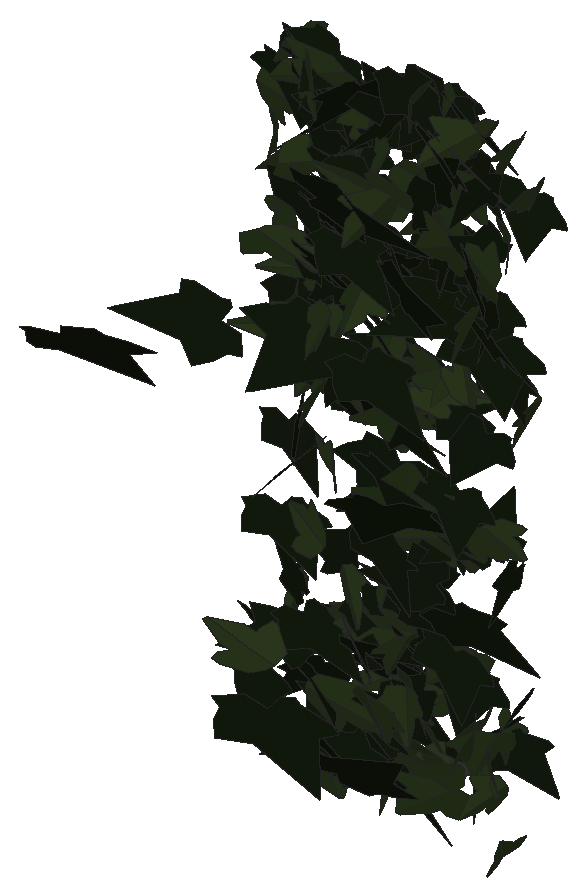
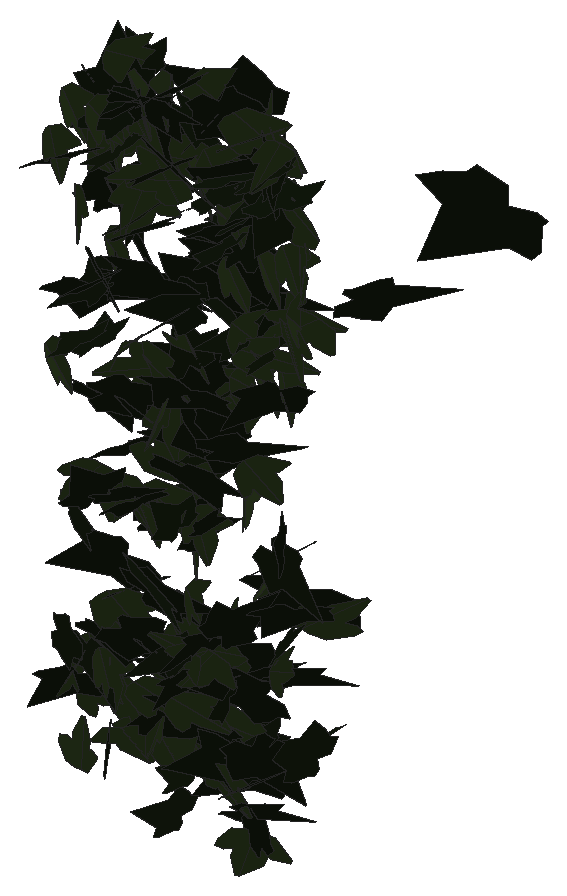
# SketchUp Ruby script. Lengths in millimetres.
U = 1.mm
M = Sketchup.active_model
def pt(a) = Geom::Point3d.new(a.map { |v| v * U })
def face(e, loops, mat)
  f = e.add_face(loops[0].map { |a| pt(a) })
  loops[1..].each { |l| e.add_face(l.map { |a| pt(a) }).erase! }
  f.material = f.back_material = mat if mat
  f
end
# faces: each face lists its corners as indices into pts; further lists are holes
def faces(e, pts, list, mat = nil) = list.each { |f| face(e, (f[0].is_a?(Array) ? f : [f]).map { |l| l.map { |i| pts[i] } }, mat) }
# xy, xz, yz: faces in a plane at the given z, y or x. An outline is a flat list of corners, or four numbers for a rectangle; further outlines are holes
def ring(l) = l.size == 4 ? [[l[0], l[1]], [l[2], l[1]], [l[2], l[3]], [l[0], l[3]]] : l.each_slice(2).to_a
def flat(e, list, mat, &to3) = list.each { |f| face(e, (f[0].is_a?(Array) ? f : [f]).map { |l| ring(l).map { |u, v| to3.(u, v) } }, mat) }
def xy(e, z, list, mat = nil) = flat(e, list, mat) { |x, y| [x, y, z] }
def xz(e, y, list, mat = nil) = flat(e, list, mat) { |x, z| [x, y, z] }
def yz(e, x, list, mat = nil) = flat(e, list, mat) { |y, z| [x, y, z] }
def lines(e, pts, list) = list.each { |a, b| e.add_line(pt(pts[a]), pt(pts[b])) }
# prism: a flat outline (further loops are holes) pulled along v
def prism(e, loops, v, mat = nil)
  f = face(e, loops, mat); d = Geom::Vector3d.new(v.map { |x| x * U })
  f.pushpull(f.normal.samedirection?(d) ? d.length : -d.length)
end
def box(e, o, s, mat = nil) = prism(e, [[o, [o[0] + s[0], o[1], o[2]], [o[0] + s[0], o[1] + s[1], o[2]], [o[0], o[1] + s[1], o[2]]]], [0, 0, s[2]], mat)
def at(x, y, z, deg = 0) = Geom::Transformation.translation(pt([x, y, z])) * Geom::Transformation.rotation(ORIGIN, Z_AXIS, deg.degrees)
def axes(o, x, y, z) = Geom::Transformation.new([*x, 0, *y, 0, *z, 0, *pt(o).to_a, 1])
def part(name) = M.definitions.add(name)
# library, detail: a bought-in or finely detailed component or shape, given as its bounding box
def library(name, o, s) = part(name).tap { |d| box(d.entities, o, s) }
def detail(e, o, s) = box(e.add_group.entities, o, s)
def put(e, d, t, mat = nil) = e.add_instance(d, t).tap { |i| i.material = mat if mat }
def group(e, t, mat = nil) = e.add_group.tap { |g| g.transformation = t; g.material = mat if mat }.entities
root = M.entities
M.materials.add("efeu1").color = [18, 25, 13]
M.materials.add("efeu2").color = [43, 57, 29]
c1 = part("ivyleaf_9")
p = [[39.1,54.8,31.7],[34.5,51.8,30.2],[-5.3,25.2,17.3],[-17.9,28.3,20.9],[-21.6,21.7,17],[-20.2,4.3,5.3],
  [-22.9,-0.3,2.5],[-17.1,-4,-0.6],[-2,-2.1,-1.2],[-0.7,-15.4,-10.1],[16.6,-22.3,-16.7],[21.1,-15.1,-12.5],
  [32.7,-10.7,-11],[46.1,-1.8,-6.6],[30.8,11.2,3.8]]
faces(c1.entities,p,[[0,1,2,3,4,5,6,7,8,9,10,11,12,13,14]],"efeu1")
c2 = part("ivyleaf_10")
p = [[0,12.8,-0.8],[-1.5,51.3,-10.9],[-4.9,51,-11.6],[-13.6,26.5,-7.3],[-13.2,15.9,-4.6],[-21.1,19.3,-7.2],
  [-29.5,16.3,-8.3],[-29.2,8.3,-6.2],[-19.7,-9.8,0.5],[-7.6,-13,4],[1,-12.2,5.8],[-0.4,51.1,-11.1],
  [-1.5,51.1,-10.9],[1,-12.4,5.9],[16.9,-12.4,3.5],[35.1,9.1,-5.1],[35,12.9,-6.1],[20.5,16.4,-4.9],
  [15.8,15,-3.8],[15.3,27.6,-7.1],[12.8,31.3,-7.8]]
faces(c2.entities,p,[[0,1,2,3,4,5,6,7,8,9,10],[11,12,0,13,14,15,16,17,18,19,20]],"efeu2")
put(root,c1,axes([3084.9,440.1,2359.8],[2.43652,0.60227,0.19081],[0.32002,0.09079,-1.41477],[-1.15902,1.29117,0.01048]))
put(root,c1,axes([3253.2,607.2,1847],[-0.95084,-0.69607,-0.93578],[1.0768,0.74556,-0.85664],[1.94097,-0.75461,0.01683]))
put(root,c1,axes([3139.5,650.3,2307],[-0.43713,-0.83768,-0.9062],[-0.15243,-0.9097,0.86121],[-2.34372,0.2154,0.11301]))
put(root,c1,axes([3401,666.2,2424.2],[0.21234,-0.26339,1.12095],[0.68031,-1.06264,-0.28526],[2.08323,0.37387,-0.0211]))
put(root,c1,axes([3288.6,659,2515.6],[1.23779,-0.49363,1.04714],[1.54799,-0.65984,-0.81622],[1.56783,1.04121,-0.02082]))
put(root,c2,axes([3362.4,672.8,2529.3],[-0.43007,-0.85809,0.7892],[0.0085,-0.80451,-0.87347],[2.21879,-0.16325,0.15632]))
put(root,c1,axes([3380.9,659.5,2140.2],[1.09267,0.78644,-0.62157],[-0.71114,-0.49678,-0.97368],[-1.7703,0.68496,0.00748]))
put(root,c1,axes([3299.5,679.7,1749.2],[2.29067,0.26504,-0.0966],[0.16641,0.05198,1.23201],[0.51044,-1.20634,0.03186]))
put(root,c2,axes([3175.6,683.9,1862.2],[0.67109,0.79349,0.70985],[-0.634,-0.628,0.86747],[1.92454,-0.48357,0.03824]))
put(root,c1,axes([3340.4,677.1,2306],[0.14442,-0.8753,-0.73036],[0.10422,0.73393,-0.87389],[2.16712,0.02304,0.0907]))
put(root,c1,axes([3302.2,682.8,2456.8],[0.32635,-0.95084,-0.60499],[-0.13617,0.60154,-0.96569],[2.14057,0.18323,0.03081]))
put(root,c2,axes([3265.3,688.2,2334.5],[0.98608,-1.04399,-0.01718],[-0.01274,0.01586,-1.16548],[1.98715,0.51816,0.00105]))
put(root,c1,axes([3257,706.1,2301.3],[-2.32839,-0.5287,0.1001],[-0.16005,-0.0577,-1.33262],[1.01152,-1.22614,0.01955]))
put(root,c2,axes([3216.5,722.5,2294.8],[0.46106,0.07581,-1.10045],[-1.9081,-0.4547,-0.25203],[-0.87544,1.03098,-0.03024]))
put(root,c2,axes([3227.8,728.4,2215.6],[0.4675,-1.1153,0.05987],[0.00274,-0.06099,-1.14197],[2.12569,0.24536,-0.0117]))
put(root,c1,axes([3392,747.8,2574.5],[-0.037,-0.57224,0.85225],[0.31829,-0.84278,-0.56207],[1.92762,0.12817,0.10917]))
put(root,c1,axes([3305.3,745.4,2033.4],[0.28687,-1.09674,0.2171],[0.11462,-0.21078,-1.10663],[2.12472,0.15945,0.03039]))
put(root,c2,axes([3281.5,742.7,2351.7],[0.43735,0.77284,-0.59729],[-0.4549,-0.55045,-0.80419],[-1.80243,0.32645,0.05803]))
put(root,c2,axes([3421.7,726,2470.2],[-1.05772,0.28526,0.81128],[-1.46021,0.27184,-0.62117],[-0.73928,-0.94506,0.0662]))
put(root,c1,axes([3388.1,745.4,2535.1],[-0.29941,0.45568,0.90404],[0.1623,-0.90567,0.47135],[1.91993,0.14762,0.10114]))
put(root,c1,axes([3440.8,755.8,2408.1],[-0.42729,0.1807,1.00874],[-0.3584,-1.02236,0.14123],[1.91719,-0.15084,0.25123]))
put(root,c1,axes([3168.2,753.6,2452.7],[0.57952,-1.00657,0.18188],[0.07841,-0.17754,-1.05155],[1.94514,0.30705,-0.0118]))
put(root,c2,axes([3414.6,763.7,2595.5],[-0.43005,-0.41598,0.99444],[-0.14831,-1.00709,-0.43898],[2.04616,-0.16043,0.17719]))
put(root,c2,axes([3315.3,751,2482.2],[-0.56727,0.07463,-1.10758],[-2.0923,0.13924,0.30523],[0.29308,1.1385,0.03528]))
put(root,c1,axes([3208.5,766.7,1710.9],[1.70196,-0.66762,-0.15371],[0.27114,-0.066,1.11553],[-1.27536,-0.90497,0.03204]))
put(root,c1,axes([3408.9,772.5,2553.5],[1.72321,-0.64183,-0.32418],[0.50025,-0.18977,1.10984],[-1.2738,-0.94281,-0.0027]))
put(root,c1,axes([3361.2,773.6,1981.8],[-0.52982,-0.10978,0.97763],[-1.44305,-0.62342,-0.28591],[1.19296,-0.80287,0.08833]))
put(root,c1,axes([3303.7,782.9,2087.5],[-0.72654,-0.62867,0.8567],[0.29997,-0.93373,-0.61496],[2,-0.08833,0.40345]))
put(root,c1,axes([3222.7,760.2,2394.3],[1.22867,-0.77965,-0.32909],[-0.29418,0.29831,-1.00997],[1.5835,0.66037,0.06771]))
put(root,c1,axes([3154.6,776.4,1838.7],[-1.21132,-0.29447,0.5931],[-0.9294,-0.34687,-0.69626],[0.85116,-0.79783,0.0838]))
put(root,c2,axes([3287.1,757.9,1803.1],[-1.50348,0.50222,0.00553],[-0.00919,0.0027,-0.9361],[-0.95584,-0.78999,0.00031]))
put(root,c1,axes([3216,782.5,2221.8],[-0.21759,-0.75041,0.67425],[-0.26801,-0.66005,-0.75848],[1.90119,-0.17893,-0.02976]))
put(root,c1,axes([3195,766,2422.5],[1.62596,-0.61914,0.39765],[0.6118,-0.23407,-1.05509],[1.25974,0.91281,-0.00084]))
put(root,c2,axes([3304.7,777.7,1715.9],[0.39413,-0.85,0.63633],[0.46084,-0.59343,-0.8715],[1.96756,0.30926,0.07665]))
put(root,c2,axes([3466.3,749.9,2432.6],[0.26733,-0.01361,1.16168],[-1.89132,0.60472,0.12725],[-1.14532,-1.00178,0.06103]))
put(root,c2,axes([3166.8,783.1,2592.8],[0.50539,-0.51544,0.98689],[1.33139,-0.71205,-0.56012],[1.64849,0.7331,0.14983]))
put(root,c1,axes([3440.1,776.5,2549.4],[-1.52417,0.39954,-0.55784],[0.96461,-0.2335,-0.89485],[-0.88029,-0.94764,-0.0147]))
put(root,c2,axes([3165.2,752.1,2483.1],[-0.21986,-0.19847,-1.04461],[1.00364,0.90173,-0.22964],[1.75725,-0.53985,0.00046]))
put(root,c2,axes([3425.5,762.8,1808.3],[0.22232,-1.01962,-0.54688],[0.076,0.55289,-1.02229],[2.20074,0.08391,0.09055]))
put(root,c1,axes([3098.4,777.6,1769.3],[0.54312,-1.01097,-0.18089],[-0.10777,0.17197,-1.05044],[1.95166,0.29083,-0.00766]))
put(root,c2,axes([3407.4,785.3,2345.9],[0.45786,-0.90348,0.49968],[0.32991,-0.47043,-0.93406],[1.93707,0.29368,0.04098]))
put(root,c2,axes([3439.1,792,1726.4],[-0.17974,-0.43705,0.83311],[0.02416,-0.83781,-0.43807],[1.79035,-0.03257,0.08955]))
put(root,c2,axes([3314.9,781.7,2071.8],[-1.7452,-0.72204,-0.07403],[-0.09923,-0.05344,1.1671],[-1.37783,0.91841,0.00971]))
put(root,c2,axes([3307,785.8,1805.3],[1.34395,-0.52767,0.49458],[0.78825,-0.27161,-0.88113],[1.12838,0.81822,0.02646]))
put(root,c1,axes([3244.7,780.8,2595],[-0.18118,0.85584,-0.73902],[0.19821,-0.73185,-0.86094],[-2.14291,-0.14005,-0.01715]))
put(root,c1,axes([3379.5,793,1886.3],[-0.28206,-1.05499,0.11095],[-0.02671,-0.11006,-1.06535],[2.01876,-0.14886,0.00141]))
put(root,c1,axes([3332,778.4,2465],[-0.32771,0.88675,0.7018],[0.03308,-0.70773,0.89851],[2.152,0.14591,0.09306]))
put(root,c1,axes([3195.2,785.2,2481.5],[0.9286,-0.87105,-0.11834],[-0.13547,0.09576,-0.99828],[1.66752,0.49285,-0.0152]))
put(root,c2,axes([3196.2,790.5,2214.6],[-0.90808,0.53739,-0.87193],[0.99316,-0.70014,-0.71707],[-1.67733,-0.70549,0.04747]))
put(root,c1,axes([3245.6,800.3,2470.5],[-0.59075,-0.90416,0.41479],[-0.0921,-0.42027,-0.95233],[1.89099,-0.30293,0.0832]))
put(root,c2,axes([3363.2,784.5,1698.1],[-1.42772,-0.2958,0.61772],[-1.04918,-0.28289,-0.80493],[0.77351,-0.92968,0.04838]))
put(root,c1,axes([3169.8,789.2,2336.5],[1.24488,-0.61005,0.54218],[0.73378,-0.38144,-0.89432],[1.36907,0.75915,-0.01367]))
put(root,c2,axes([3358.5,786.3,1708.8],[-1.74347,0.04496,0.43505],[0.82771,-0.01342,0.91715],[0.08826,1.01404,-0.00715]))
put(root,c1,axes([3295.8,788.6,2572.2],[-1.1846,0.63623,-0.49306],[0.47977,-0.43784,-0.88321],[-1.45486,-0.66243,0.11021]))
put(root,c1,axes([3419.2,800.5,2415.6],[0.00324,0.11962,1.08392],[-1.59034,-0.69631,0.07815],[1.33353,-0.83069,0.09057]))
put(root,c2,axes([3384.4,785.4,2522.4],[-1.95028,0.14394,-0.2906],[0.54453,-0.0521,-1.03473],[-0.29054,-1.06387,0.01136]))
put(root,c2,axes([3431.6,792.6,1791.2],[-0.86257,-0.9324,0.17488],[-0.08647,-0.17226,-1.03616],[1.80342,-0.45422,0.03396]))
put(root,c1,axes([3270.9,809.1,2243.7],[-0.18269,-0.54405,0.96814],[0.39272,-0.96357,-0.52102],[2.07677,0.13435,0.18369]))
put(root,c2,axes([3407.8,801.6,1763],[0.71613,-0.38277,0.77565],[1.24941,-0.42438,-0.52789],[1.07185,0.75041,0.09711]))
put(root,c1,axes([3373.9,805.7,2092.7],[-0.43802,-0.99245,0.12721],[-0.05686,-0.12366,-1.01878],[1.90343,-0.23208,-0.00116]))
put(root,c2,axes([3443.8,804.8,1638],[-0.29026,-0.70602,-0.60976],[-0.04532,-0.6147,0.7177],[-1.77488,0.13116,0.08139]))
put(root,c2,axes([3337.6,791.6,2026.4],[-1.19599,-0.13183,0.94599],[-1.76374,-0.18997,-0.64208],[0.44005,-1.11969,-0.00244]))
put(root,c1,axes([3256.8,804,1696.5],[-0.74716,-0.77052,-0.50341],[-0.40922,-0.45537,0.86467],[-1.70322,0.44741,0.01309]))
put(root,c1,axes([3386.1,770.9,2408.6],[-0.30052,0.36324,-1.00284],[-1.44779,0.67224,0.36327],[1.42287,0.76073,0.15783]))
put(root,c2,axes([3166,798.1,1964.2],[-0.46675,1.02137,0.39064],[0.13226,-0.38497,1.0502],[2.07699,0.25404,0.02091]))
put(root,c2,axes([3193.2,797.6,2591.1],[-1.20065,-0.1592,0.89678],[-1.61173,-0.29902,-0.64882],[0.63806,-1.05489,0.04858]))
put(root,c1,axes([3324.5,799.9,1815.1],[-1.51212,0.38254,-0.44095],[0.76247,-0.18434,-0.88178],[-0.80807,-0.88978,-0.00689]))
put(root,c2,axes([3181.3,801.3,1758.5],[-0.3134,0.10605,-1.11198],[1.91133,-0.47807,-0.19431],[-0.9308,-1.01739,-0.02461]))
put(root,c2,axes([3106,790.2,2345.3],[-1.27581,-0.33147,-0.64256],[1.18156,0.18523,-0.74323],[0.70529,-0.90991,0.08278]))
put(root,c1,axes([3192.7,810.1,2415.3],[1.31726,-0.80626,0.01305],[0.00302,0.01856,1.06251],[-1.53467,-0.692,0.01329]))
put(root,c1,axes([3367.6,808.8,2330.7],[-1.84984,-0.29067,0.36021],[-0.6622,-0.09369,-1.01445],[0.58095,-1.03232,-0.00936]))
put(root,c1,axes([3155.5,797.2,1856.5],[0.39308,-0.86307,-0.53471],[0.16101,0.5584,-0.86862],[1.92557,0.12949,0.18179]))
put(root,c1,axes([3230.8,806.9,2351.8],[1.78503,-0.05542,0.63483],[-1.20769,0.02244,0.93946],[-0.11129,-1.13233,-0.01245]))
put(root,c2,axes([3273,797.8,2236.5],[1.56309,-0.66676,0.03168],[-0.00802,0.04505,1.05738],[-1.27037,-0.82067,0.0323]))
put(root,c1,axes([3255.2,820.6,2559.6],[-0.49584,-0.15666,1.01123],[-0.73627,-0.95097,-0.24699],[1.80299,-0.43142,0.17724]))
put(root,c1,axes([3382.1,795.7,1933.9],[-0.15104,-0.03443,-0.9948],[1.43443,0.64979,-0.08262],[1.23746,-0.75743,-0.02565]))
put(root,c1,axes([3268,810.2,2162.9],[0.15789,-0.19874,-1.04068],[2.01641,0.01867,0.08089],[0.00601,-1.04382,0.19959]))
put(root,c1,axes([3207.9,800.6,2398.9],[-0.68409,-0.27514,-1.03314],[1.57543,0.61821,-0.45263],[1.28782,-0.90244,0.00492]))
put(root,c1,axes([3278.1,811.6,2096.2],[-1.85879,-0.30246,-0.28557],[0.51789,0.08665,-1.02243],[0.59878,-1.01386,-0.00219]))
put(root,c1,axes([3156.3,820.6,1760.7],[0.08444,-0.68309,0.67983],[0.18445,-0.67394,-0.68349],[1.82488,0.09973,0.03763]))
put(root,c2,axes([3290.2,807.9,1864.8],[-0.2608,-0.89487,0.15217],[0.00736,-0.15447,-0.9049],[1.72754,-0.13444,0.02683]))
put(root,c1,axes([3295.5,806.1,2610.4],[0.49292,-1.03557,-0.41472],[-0.11935,0.41156,-1.06684],[2.1197,0.26399,0.03637]))
put(root,c2,axes([3211.4,806.8,2483.5],[-0.19005,-1.03888,0.04189],[0.00666,-0.04242,-1.04364],[1.97879,-0.09963,0.00754]))
put(root,c2,axes([3322.3,788.1,2597.2],[-0.00405,0.70633,0.73753],[-0.9191,0.64916,-0.62308],[-1.71249,-0.35008,0.33267]))
put(root,c2,axes([3380.7,811.2,1875.4],[-1.11229,-0.66081,0.51555],[-0.65527,-0.38374,-0.88217],[1.45432,-0.6783,-0.00317]))
put(root,c1,axes([3141.6,801.4,1888],[-0.25727,-0.68569,0.59126],[0.23223,0.57856,0.69886],[-1.70745,0.18201,0.00596]))
put(root,c2,axes([3275.2,795.5,2009],[0.67239,-0.86472,-0.61308],[-0.08643,0.6333,-0.9194],[2.01554,0.31563,0.1651]))
put(root,c2,axes([3129.2,802,2267],[0.18738,-0.9927,-0.27687],[0.04652,0.2803,-0.99631],[1.96087,0.08821,0.05009]))
put(root,c2,axes([3186.9,821.7,2253.7],[-0.007,-0.60279,0.81926],[0.57289,-0.78321,-0.57491],[1.84908,0.24038,0.18122]))
put(root,c2,axes([3282,814.4,1803.6],[0.36659,-0.27309,0.86289],[1.53083,-0.35283,-0.29121],[0.78976,0.81067,0.16394]))
put(root,c2,axes([3206.9,810,2393.9],[-0.10409,-1.02546,0.1331],[-0.02027,-0.13272,-1.02691],[1.96791,-0.05561,-0.00354]))
put(root,c1,axes([3204.8,788.3,2307.9],[-0.92227,1.0072,-0.10852],[-0.12772,0.08812,1.11749],[1.92377,0.48871,0.02216]))
put(root,c2,axes([3261.8,806.8,2504.4],[0.65276,-0.93518,-0.14007],[-0.10004,0.12991,-0.99608],[1.7969,0.34695,-0.00458]))
put(root,c2,axes([3338.6,809.5,2016.7],[1.47176,-0.51798,0.01839],[0.03125,-0.00854,-0.93075],[0.98594,0.77348,0.00205]))
put(root,c1,axes([3419.6,814.1,2300.3],[-0.92838,-0.88386,-0.4176],[0.3419,0.3777,-1.00927],[1.82878,-0.51931,-0.02331]))
put(root,c2,axes([3124.8,824,1875.6],[-0.02215,-0.42153,0.86806],[0.58765,-0.82411,-0.39604],[1.74003,0.27296,0.1448]))
put(root,c2,axes([3390.4,804.8,2036.4],[-1.74365,-0.23142,0.04825],[-0.08761,-0.01476,-0.94494],[0.44129,-0.91732,0.00303]))
put(root,c1,axes([3376.1,823.6,2032.4],[-1.26923,-0.54566,0.43347],[-0.57695,-0.31309,-0.8605],[1.19424,-0.73118,0.04497]))
put(root,c2,axes([3288,805.6,2163.8],[-1.51013,-0.70618,-0.08184],[0.11621,0.05449,-1.06221],[1.348,-0.79582,-0.00011]))
put(root,c2,axes([3208.4,809.8,1918.9],[-0.19134,1.00304,-0.28661],[0.06129,-0.28482,-1.00806],[-1.98445,-0.10551,-0.0035]))
put(root,c1,axes([3341.9,812.8,2374.8],[-0.20529,0.66897,0.83861],[0.22888,-0.82998,0.67756],[2.02878,0.16133,0.00842]))
put(root,c2,axes([3195.9,789.8,2070.8],[0.41272,0.00371,-0.98074],[-0.28565,0.99272,-0.02944],[1.84456,0.15291,0.21488]))
put(root,c1,axes([3207.1,808.1,2154.7],[1.60581,-0.27506,0.55498],[0.98486,-0.20238,-0.88703],[0.64786,0.98942,-0.02715]))
put(root,c2,axes([3231.6,819,2539.9],[-0.30495,-0.92843,0.35833],[0.30006,-0.38205,-0.91937],[1.8701,-0.0901,0.20594]))
put(root,c2,axes([3390.4,806.4,2528.8],[0.03382,-0.94548,-0.37206],[-0.03605,0.37174,-0.94558],[1.93341,0.02347,-0.01112]))
put(root,c1,axes([3173.2,833.3,2590],[-0.89668,-0.69278,0.63141],[-0.30355,-0.63713,-0.81806],[1.75794,-0.46338,0.18081]))
put(root,c1,axes([3170.9,807.1,1718.1],[-0.18251,-0.48991,-0.89341],[0.64199,0.8315,-0.49217],[1.82986,-0.34058,0.08356]))
put(root,c2,axes([3288.6,823.4,1712.2],[-1.33974,0.04576,0.86687],[1.51235,-0.41533,0.6672],[0.66509,1.03658,0.22906]))
put(root,c2,axes([3345.3,806.2,2448.8],[-1.00765,-0.8289,-0.45128],[0.47787,0.37508,-0.98352],[1.73148,-0.5859,0.00882]))
put(root,c1,axes([3168.1,824.3,2493.4],[0.69386,-1.0688,0.09804],[0.05186,-0.09429,-1.12926],[2.04202,0.36557,-0.00463]))
put(root,c2,axes([3396.9,814,1790.5],[-0.1044,-1.09654,-0.1535],[-0.007,0.15387,-1.09785],[2.10727,-0.05381,-0.01125]))
put(root,c1,axes([3431.7,804.1,1795.6],[-0.27322,0.93492,0.00845],[-0.00831,0.00788,-0.94587],[-1.7794,-0.14359,0.00312]))
put(root,c2,axes([3349,813.9,2596.4],[0.69771,-1.07233,-0.23436],[-0.09631,0.23031,-1.13297],[2.08682,0.36916,0.02607]))
put(root,c1,axes([3331.5,819.6,2432.4],[0.63617,-0.93672,-0.22513],[-0.12064,0.2164,-0.99449],[1.82956,0.33998,0.01271]))
put(root,c1,axes([3221.1,814.6,1821],[1.0526,-0.19838,0.69335],[1.25841,-0.20934,-0.58733],[0.54795,0.86185,0.01693]))
put(root,c1,axes([3148.3,793.3,2493.1],[0.49843,0.88766,0.62906],[0.34895,0.60177,-0.92548],[-2.041,0.31966,-0.00461]))
put(root,c2,axes([3300.4,811.2,2484.6],[0.86907,-0.13516,0.8889],[1.60249,0.41397,-0.36959],[-0.60021,0.90956,0.30031]))
put(root,c2,axes([3111.5,818.8,2447],[-0.18858,-1.0426,0.00152],[-0.00076,-0.00149,-1.0473],[1.98428,-0.09909,-0.00026]))
put(root,c1,axes([3396.5,815.6,2320.6],[1.3985,-0.73887,-0.29181],[-0.36794,0.21923,-1.04192],[1.46647,0.75964,0.01686]))
put(root,c1,axes([3204,827.6,2430.3],[0.52137,-0.94111,0.13728],[0.06473,-0.13307,-0.98016],[1.80891,0.27601,-0.00449]))
put(root,c1,axes([3378.9,825.2,1840.3],[-1.48229,-0.29801,-0.42666],[0.79017,0.10725,-0.8328],[0.59722,-0.88154,0.04291]))
put(root,c1,axes([3128,820.9,2524.9],[-0.0591,0.78078,0.7162],[-0.49239,-0.70041,0.75234],[1.95542,-0.15277,0.21109]))
put(root,c1,axes([3100.9,821.7,1968.5],[-0.35709,-0.85694,-0.49129],[0.31095,0.46627,-0.87568],[1.85405,-0.24324,0.05224]))
put(root,c2,axes([3159.7,830.6,2303.6],[-0.33416,-0.04246,1.0018],[-1.26673,-0.75573,-0.14868],[1.42728,-0.68066,0.10259]))
put(root,c1,axes([3174.5,824,2321.1],[1.07258,-0.89168,-0.02546],[-0.02582,0.02154,-1.05485],[1.69755,0.56373,0.00004]))
put(root,c2,axes([3251.5,830.1,1939.5],[0.14587,-0.86137,0.41055],[0.44851,-0.38203,-0.84552],[1.75979,0.16877,0.18146]))
put(root,c1,axes([3121,839,2549.5],[-0.34695,-0.08431,1.02203],[-0.29141,-1.02417,-0.1118],[1.92985,-0.16981,0.16686]))
put(root,c2,axes([3330.3,803.4,2214.6],[0.12069,0.16377,1.02197],[0.78131,0.93592,-0.17545],[-1.80826,0.41532,-0.0076]))
put(root,c1,axes([3236.3,840.2,2037.8],[0.0735,-0.40126,-0.83176],[0.6187,-0.77329,0.38814],[-1.64508,-0.30876,0.10882]))
put(root,c1,axes([3106,843.6,2531.5],[-0.53746,-0.87158,0.69569],[0.38782,-0.7459,-0.85177],[2.0867,-0.08586,0.33749]))
put(root,c1,axes([3393.1,829.5,2166.3],[-1.66602,-0.18721,-0.30549],[0.58207,0.02968,-0.89456],[0.35521,-0.92668,0.03307]))
put(root,c2,axes([3332.2,811.8,2230.7],[0.60863,-0.35302,-0.91849],[-1.26106,0.63674,-0.47543],[1.38451,0.73515,-0.02927]))
put(root,c1,axes([3395,830.4,2338.4],[-1.03887,0.22324,-0.80192],[1.41145,-0.30508,-0.58974],[-0.71947,-0.92084,0.00097]))
put(root,c1,axes([3171.5,835.5,1673.9],[-1.2193,-0.27348,0.56649],[-0.89939,-0.32443,-0.69106],[0.79018,-0.79126,0.08756]))
put(root,c1,axes([3433.4,834.3,1995.8],[-0.95952,0.11978,-0.79649],[1.23073,-0.49999,-0.48452],[-0.91388,-0.79911,0.18376]))
put(root,c1,axes([3189.3,838.6,1825.7],[0.65743,-0.26956,-0.91918],[1.53586,-0.44453,0.43363],[-0.98217,-0.87556,0.06282]))
put(root,c1,axes([3131.8,826.8,2314.9],[0.90402,-0.85088,-0.08182],[-0.06443,0.07481,-0.97446],[1.6256,0.47615,0.00688]))
put(root,c1,axes([3330.1,816.5,1910.3],[-0.37952,0.13422,0.89928],[-1.32055,0.57251,-0.23931],[-1.11832,-0.72159,-0.02259]))
put(root,c1,axes([3330.3,832.8,2591.3],[-1.7951,-0.36605,-0.14838],[0.24788,0.07443,-1.0115],[0.70969,-0.95189,-0.02203]))
put(root,c2,axes([3068.4,838.2,2509.8],[0.24193,-0.18077,-1.02809],[1.15253,-0.83082,0.22096],[-1.6182,-0.61876,0.00367]))
put(root,c1,axes([3348.2,835.5,1860.9],[-0.29446,-0.05646,-0.93104],[-0.72104,-0.8586,0.11503],[-1.62218,0.39189,0.11788]))
put(root,c2,axes([3409.9,817.8,2048.7],[-1.052,-0.54128,-0.53516],[0.82601,0.3192,-0.77114],[1.19008,-0.70003,0.06216]))
put(root,c1,axes([3329,846,2418.9],[-0.88925,-0.678,0.58718],[-0.41394,-0.55666,-0.81584],[1.65607,-0.5032,0.11137]))
put(root,c2,axes([3222.7,835.9,1858.9],[-0.8667,-0.45054,0.6455],[-0.64212,-0.56205,-0.63032],[1.35359,-0.55511,0.1143]))
put(root,c1,axes([3240.7,838.7,1705.4],[0.5865,-0.97245,0.26451],[0.1666,-0.24973,-1.02008],[1.91077,0.32026,0.00775]))
put(root,c2,axes([3090.5,818.6,2470.4],[0.55522,-0.86162,-0.5234],[0.06321,0.55279,-0.89149],[1.91764,0.23125,0.18093]))
put(root,c1,axes([3194.8,848.7,2507.9],[-0.57682,-0.60694,0.7858],[0.12528,-0.83207,-0.61729],[1.88554,-0.13039,0.28141]))
put(root,c1,axes([3333.6,836.7,2043.4],[-0.16078,-0.91933,-0.11123],[-0.00061,0.11172,-0.92315],[1.76243,-0.08383,-0.01046]))
put(root,c2,axes([3242.4,829.2,2047.7],[-0.40734,-1.02754,-0.02071],[0.00967,0.0201,-1.04959],[1.95598,-0.21409,0.00087]))
put(root,c1,axes([3204.3,839.4,2158.8],[-0.75299,0.02717,0.90439],[-1.62852,-0.33206,-0.36436],[0.55969,-0.92962,0.15658]))
put(root,c2,axes([3208.5,822.8,1850.5],[-0.67728,-0.23953,1.03534],[1.77455,0.45346,0.42539],[-0.97033,0.99647,0.05529]))
put(root,c1,axes([3246.9,823,1769.4],[-0.16104,-0.32364,-1.03938],[1.21496,0.8297,-0.31032],[1.6782,-0.63173,0.12492]))
put(root,c2,axes([3312.7,837.5,1789.6],[-0.8388,-0.23806,0.79955],[-1.16422,-0.52263,-0.49281],[1.07956,-0.74859,0.08978]))
put(root,c1,axes([3370.2,843.3,2180.3],[-1.00772,-0.5655,-0.666],[-0.41129,-0.66979,0.74053],[-1.61116,0.52468,0.22752]))
put(root,c1,axes([3326.5,834.2,2588.8],[-0.05976,-0.92521,-0.4228],[-0.03628,0.42347,-0.92524],[1.93567,-0.02063,-0.0304]))
put(root,c2,axes([3385.1,843.1,2561.8],[0.03662,-0.88876,0.53137],[0.07127,-0.53052,-0.88869],[1.96946,0.03572,0.02228]))
put(root,c1,axes([3176.2,847.4,2544.9],[-0.20729,-0.96056,0.28969],[0.52321,-0.30881,-0.9206],[1.83638,-0.02044,0.29499]))
put(root,c2,axes([3372.8,816.9,2220.4],[0.13293,0.83129,-0.62397],[-0.16993,0.62786,0.82649],[1.97091,-0.00193,0.11334]))
put(root,c2,axes([3345.8,836.6,1720.7],[1.31758,0.48876,-0.3775],[-0.56892,-0.23103,-0.84731],[-1.02851,0.75393,-0.01491]))
put(root,c1,axes([3053.3,842.9,1791.8],[1.01208,-0.87396,0.39802],[0.43036,-0.32822,-1.02282],[1.77631,0.57748,0.02103]))
put(root,c1,axes([3444.4,842.1,1827.5],[-0.82545,0.30992,-0.7181],[0.85934,-0.57126,-0.51925],[-1.21544,-0.61437,0.12057]))
put(root,c1,axes([3121,834,2041.6],[-0.83566,0.84469,-0.55493],[0.47339,-0.49611,-0.95197],[-1.86434,-0.50459,0.00702]))
put(root,c1,axes([3145.5,826.5,1838.7],[0.44951,-0.01945,-0.87995],[1.18814,0.64595,0.15329],[1.18084,-0.64253,0.18074]))
put(root,c1,axes([3205.9,828,2525.6],[-1.73438,-0.43775,0.27809],[0.46793,0.13037,1.01093],[-0.86905,0.94382,-0.01066]))
put(root,c2,axes([3250.2,844.6,1794],[-0.72698,-0.4071,0.73145],[-0.6589,-0.65519,-0.54546],[1.45054,-0.50165,0.11882]))
put(root,c1,axes([3189.4,845.1,2475.9],[-0.4162,-0.97219,-0.06189],[0.01441,0.06173,-0.99647],[1.85397,-0.21873,-0.00615]))
put(root,c2,axes([3432,838.2,2560.8],[0.10984,-1.0048,0.10155],[-0.00635,-0.10191,-1.00641],[1.92206,0.05709,-0.00913]))
put(root,c1,axes([3292.6,836,2361.9],[-0.62183,-0.47618,-0.97385],[1.53725,0.57143,-0.55041],[1.37601,-0.85358,0.17481]))
put(root,c1,axes([3249,839.2,2226.2],[-0.80441,-0.57459,-0.69219],[1.1068,0.40898,-0.69459],[1.30627,-0.70036,0.16227]))
put(root,c1,axes([3260.9,824.3,2326.4],[1.0291,-0.53779,-0.74074],[-0.42877,0.75567,-0.71309],[1.68856,0.51965,0.27038]))
put(root,c1,axes([3189.7,819.5,1726.4],[1.10547,0.27349,0.64911],[1.00152,0.39077,-0.63553],[-0.8911,0.77847,0.09098]))
put(root,c1,axes([3146.3,839.9,1770],[-0.04242,0.6239,-0.76266],[-0.07214,-0.76283,-0.62293],[-1.87391,0.01524,0.04125]))
put(root,c1,axes([3352.4,843.2,2519.7],[0.56659,-0.95907,-0.03031],[-0.00724,0.03056,-1.0042],[1.8262,0.29768,0.00542]))
put(root,c2,axes([3098.9,831.3,2351.8],[1.16649,-0.69917,-0.36837],[-0.1922,0.39306,-0.91405],[1.49172,0.59738,0.17029]))
put(root,c1,axes([3219.6,825,1887.1],[0.31795,-0.33779,-0.8306],[-0.18762,0.83285,-0.35853],[1.69618,0.15544,0.11604]))
put(root,c1,axes([3427.5,831.4,1768.8],[-0.12261,-0.53687,-0.74799],[0.2248,0.73881,-0.54045],[1.73783,-0.13345,0.01714]))
put(root,c1,axes([3116.8,853.5,2568.9],[0.06111,-0.95359,0.40649],[0.15783,-0.40302,-0.95199],[1.96655,0.06198,0.06377]))
put(root,c1,axes([3266.8,834.2,1857.9],[1.38053,-0.54547,-0.21984],[-0.22522,0.20656,-0.90298],[1.09639,0.72927,0.09133]))
put(root,c1,axes([3376.8,857.2,2253.5],[-0.38494,-0.61899,0.74105],[-0.02071,-0.75562,-0.63414],[1.83754,-0.13819,0.14809]))
put(root,c1,axes([3439.9,853.7,2486.2],[-0.5743,-0.95655,0.15088],[0.07003,-0.16924,-0.99941],[1.84169,-0.29185,0.08505]))
put(root,c2,axes([3158.7,854.6,2349.8],[-0.33529,-0.66482,0.74787],[0.53699,-0.76156,-0.61053],[1.82716,0.10183,0.31667]))
put(root,c1,axes([3402.9,826.4,2022.6],[-0.76134,-0.30044,0.87943],[1.2806,0.56677,0.4997],[-1.21999,0.78242,-0.02428]))
put(root,c2,axes([3208.8,834.3,1711.8],[1.17606,-0.32297,-0.59003],[-0.88745,0.37176,-0.69185],[0.92264,0.76927,0.08663]))
put(root,c2,axes([3077.9,853.9,2391.2],[0.3477,-0.60037,0.75677],[0.73177,-0.66135,-0.61749],[1.68657,0.41072,0.1119]))
put(root,c2,axes([3303.2,833,1749.8],[-1.00253,0.73649,0.16397],[-0.22301,0.1177,-0.90509],[-1.41858,-0.53899,0.02641]))
put(root,c1,axes([3362,853.4,1704.9],[-0.117,0.02149,-0.92568],[1.40548,-0.5585,-0.06201],[-1.06304,-0.74077,0.0199]))
put(root,c1,axes([3384.8,851.4,2332.9],[-0.08852,-0.98064,0.04025],[-0.01156,-0.04,-0.98174],[1.86789,-0.04672,-0.00417]))
put(root,c2,axes([3153.4,836.5,1640],[-1.39188,-0.4943,-0.20702],[0.34462,0.10172,-0.88256],[0.95994,-0.75323,0.01667]))
put(root,c1,axes([3130.7,850.7,1650.1],[-0.04887,0.14488,0.90595],[0.33998,-0.88817,0.1471],[1.71269,0.18044,-0.00335]))
put(root,c2,axes([3294.4,827.4,2179.9],[0.35857,-0.77312,-0.71532],[0.42628,0.73946,-0.74022],[1.95876,-0.0194,0.29204]))
put(root,c1,axes([3181.4,855,1922.8],[0.18156,0.07332,1.01492],[-1.52944,-0.61989,0.12032],[1.188,-0.80926,-0.00021]))
put(root,c1,axes([3148.6,859.7,1724.1],[-0.68184,-0.75572,0.52668],[-0.26071,-0.51512,-0.83231],[1.73362,-0.37469,0.08198]))
put(root,c1,axes([3237.1,842.9,2346.8],[1.45845,-0.5934,0.19678],[0.30147,-0.11684,-0.9692],[1.15101,0.7825,0.00451]))
put(root,c1,axes([3251.5,856.3,2046.7],[0.33508,-0.69879,0.57439],[0.32022,-0.54966,-0.72027],[1.69151,0.24248,0.02257]))
put(root,c2,axes([3223.2,838.6,1865.4],[-1.64448,0.08888,-0.27068],[0.51601,-0.00894,-0.86843],[-0.16653,-0.90542,-0.018]))
put(root,c1,axes([3277.5,848.7,2526],[0.19281,-0.9926,-0.20243],[0.05358,0.20612,-0.9966],[1.92725,0.09357,0.04796]))
put(root,c2,axes([3447.5,849.5,2210.7],[0.37168,-0.97298,0.24226],[0.08226,-0.23841,-0.99237],[1.90653,0.19997,-0.00441]))
put(root,c1,axes([3115.9,835.1,2269.3],[0.06843,-0.63583,-0.8599],[0.03571,0.86063,-0.63559],[2.03505,0.00628,0.04007]))
put(root,c1,axes([3340.7,845.7,2579.4],[1.27601,-0.77657,-0.01064],[-0.00394,0.01227,-1.02593],[1.4781,0.67043,0.00645]))
put(root,c2,axes([3452.9,842.4,2502.8],[-0.11415,-0.99727,-0.13968],[0.05543,0.13815,-0.99886],[1.91573,-0.06342,0.02058]))
put(root,c1,axes([3244.9,839.5,1836.8],[0.19257,-0.6731,-0.60781],[-0.21003,0.5979,-0.68049],[1.71321,0.14896,-0.0151]))
put(root,c1,axes([3298.6,837.2,2533.3],[-1.38693,0.65171,0.28984],[-0.3717,0.21621,-0.97719],[-1.30558,-0.75387,-0.0297]))
put(root,c2,axes([3138.3,854.1,2161.6],[-0.56274,-0.78757,0.49781],[-0.17179,-0.49561,-0.83769],[1.76488,-0.29936,0.07719]))
put(root,c2,axes([3426.8,826.5,1781.5],[0.29785,-0.37876,-0.92256],[0.29611,0.93169,-0.35611],[1.87479,-0.08698,0.20281]))
put(root,c1,axes([3400,859.5,2247.8],[0.0501,-0.91806,0.3378],[0.1786,-0.33399,-0.91502],[1.85318,0.05701,0.07905]))
put(root,c2,axes([3124.6,847.4,2444.8],[0.37734,-0.97173,0.0115],[0.00534,-0.01117,-0.99175],[1.84952,0.19829,0.00052]))
put(root,c1,axes([3085.7,854,2061.7],[0.2165,-1.01564,-0.05401],[-0.02334,0.05298,-1.02197],[1.93556,0.11424,-0.00628]))
put(root,c1,axes([3114,827.6,2049.5],[-0.06769,-0.10437,0.99796],[0.52496,0.9591,0.11014],[-1.83611,0.27806,-0.0053]))
put(root,c2,axes([3118.1,834.4,2594.3],[-0.56293,-0.77346,-0.63277],[0.56899,0.56119,-0.82572],[1.81479,-0.41587,0.06261]))
put(root,c2,axes([3419.4,836.6,2431.1],[0.77644,-0.76983,-0.51925],[0.03276,0.57333,-0.83648],[1.76698,0.32765,0.24368]))
put(root,c1,axes([3252.6,853.8,1648.2],[0.86728,-0.79853,0.24374],[0.20613,-0.21879,-0.9193],[1.57555,0.46819,-0.0139]))
put(root,c1,axes([3320.9,829,1937.7],[-0.38139,0.78529,0.56916],[-0.3795,0.53541,-0.80893],[-1.8064,-0.27828,0.04978]))
